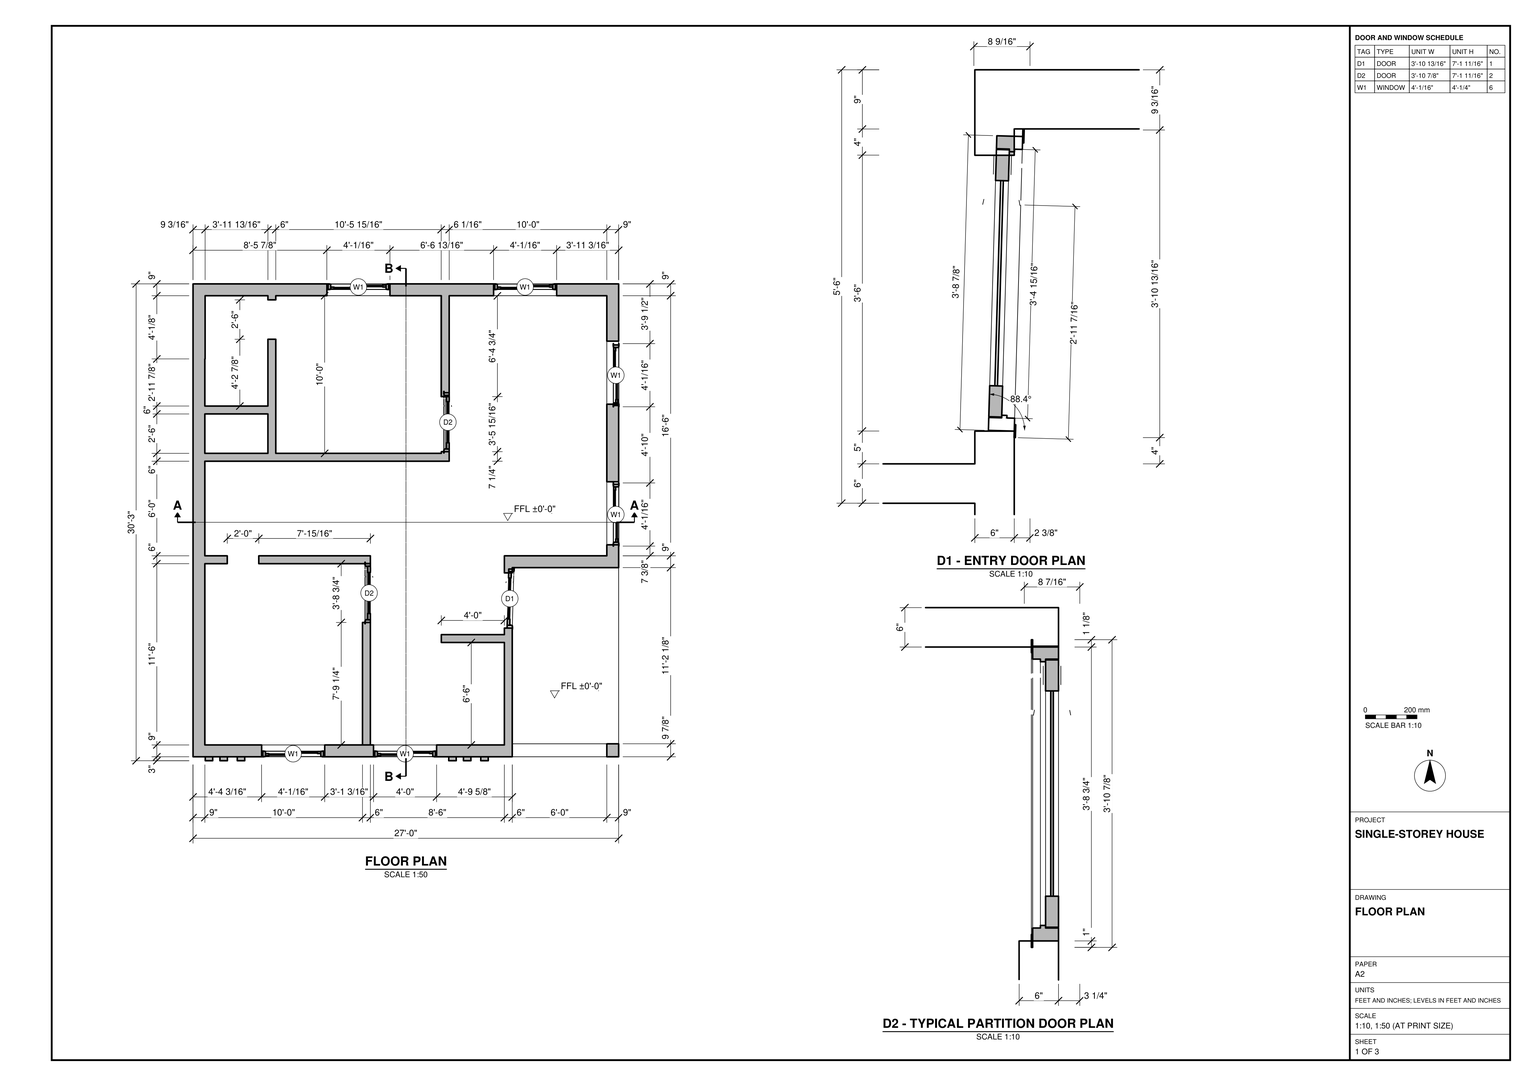
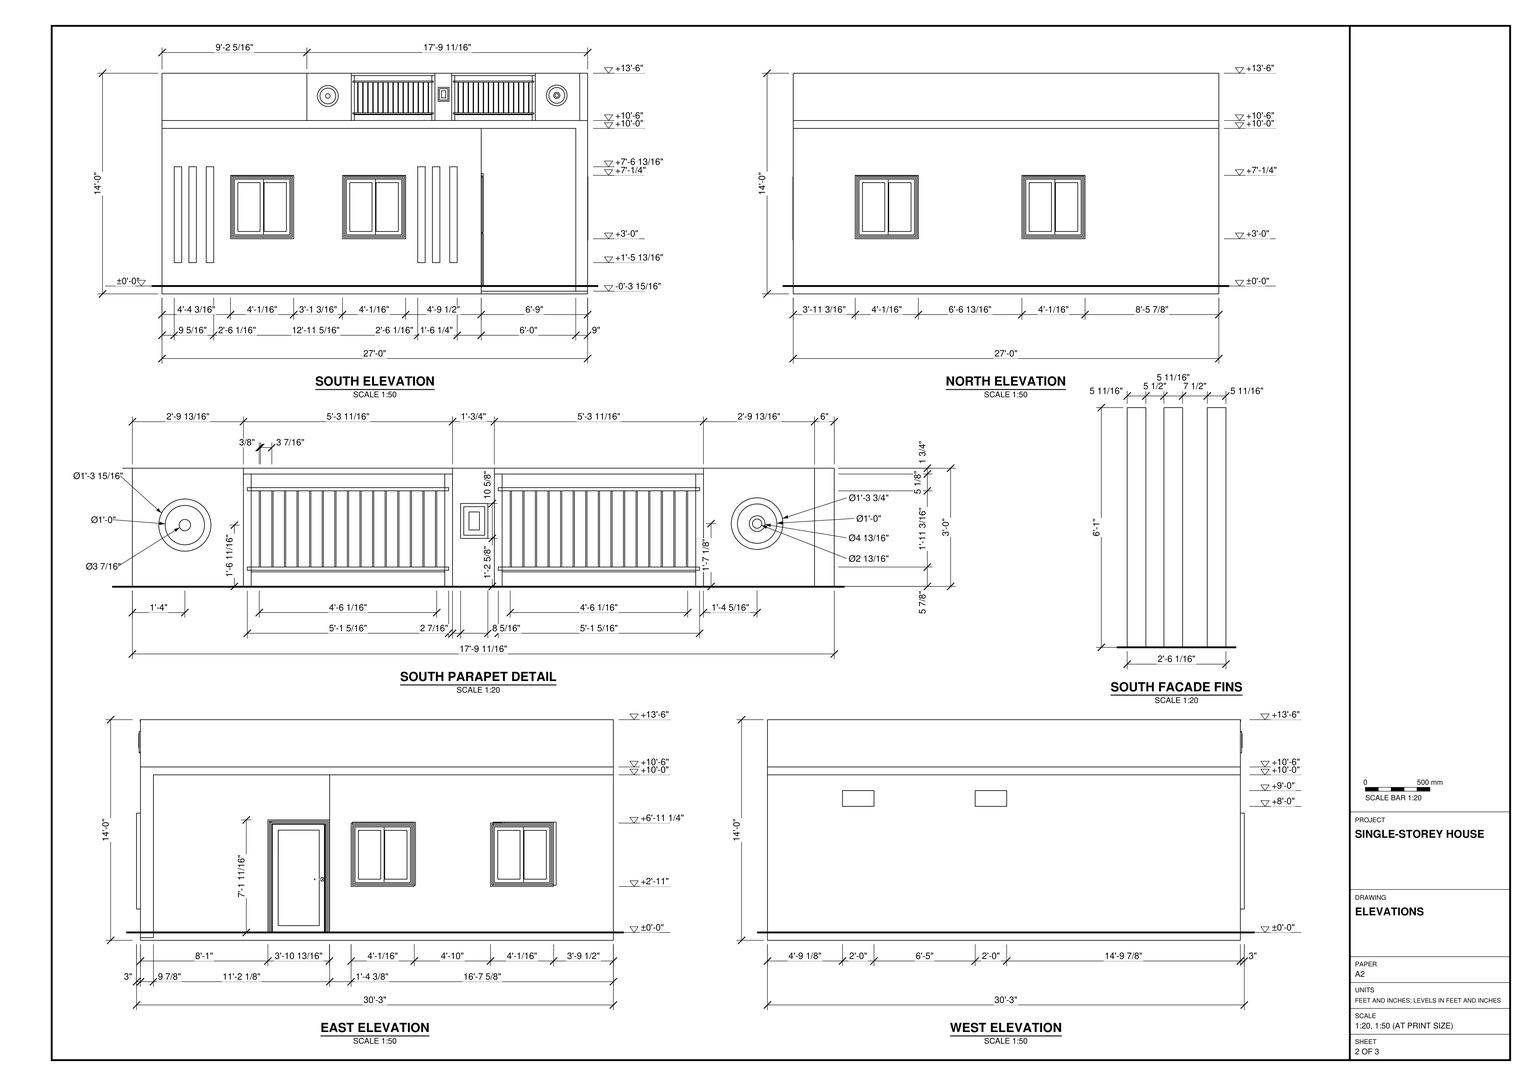
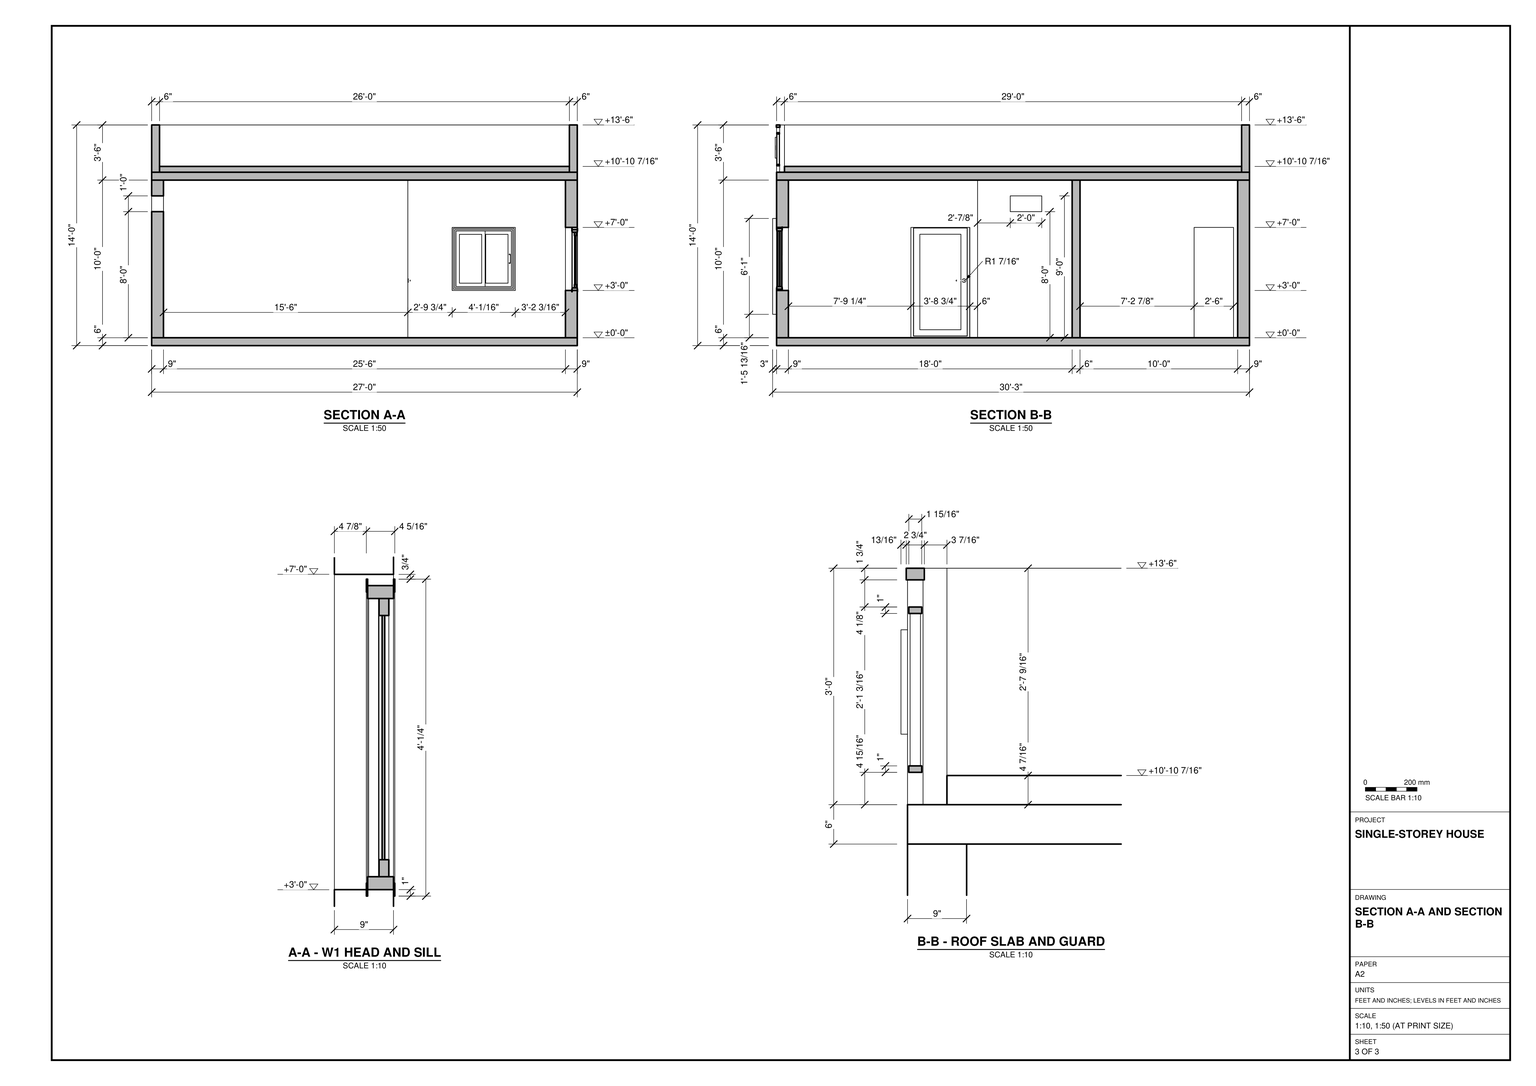
Build the single-storey house in SketchUp from task_files/diagram_01.pdf. Work in feet and inches. Set the finished floor at ±0'-0". The overall model measures 27'-3/16" east to west, 30'-3" north to south and 14'-0" from the underside of the floor slab to the top of the parapet.

Use the floor plan to set out the 9" main exterior walls and 6" partitions, following the thickness changes at the entry. Leave the southeast corner open beneath the roof, with a corner post and an entry door in the east-facing wall of the recess. Match the internal wall runs, passage gaps and two partition doors. Fit the sliding windows in pairs on the south, north and east walls, and include the two small high openings on the west wall. Use the enlarged details for the door frames, window heads and sills.

Model the floor slab, flat roof slab and perimeter parapet to the sections. On the south elevation, place the vertical fins on either side of the window pair. Above them, follow the parapet detail for the barred panels, central rectangular relief and circular end motifs. Leave the rooms unfurnished as drawn. Any decor or loose items may be suitable library components.

Keep walls, slabs and roof separate as groups or components, treat any furniture or joinery piece separately, and use components for repeated parts. Save one SketchUp model as output_files/single_storey_house_with_a_recessed_entry_and_parapet.skp.

# SketchUp Ruby script. Lengths in inches.
U = 1.inch
M = Sketchup.active_model
def pt(a) = Geom::Point3d.new(a.map { |v| v * U })
def face(e, loops, mat)
  f = e.add_face(loops[0].map { |a| pt(a) })
  loops[1..].each { |l| e.add_face(l.map { |a| pt(a) }).erase! }
  f.material = f.back_material = mat if mat
  f
end
# faces: each face lists its corners as indices into pts; further lists are holes
def faces(e, pts, list, mat = nil) = list.each { |f| face(e, (f[0].is_a?(Array) ? f : [f]).map { |l| l.map { |i| pts[i] } }, mat) }
# xy, xz, yz: faces in a plane at the given z, y or x. An outline is a flat list of corners, or four numbers for a rectangle; further outlines are holes
def ring(l) = l.size == 4 ? [[l[0], l[1]], [l[2], l[1]], [l[2], l[3]], [l[0], l[3]]] : l.each_slice(2).to_a
def flat(e, list, mat, &to3) = list.each { |f| face(e, (f[0].is_a?(Array) ? f : [f]).map { |l| ring(l).map { |u, v| to3.(u, v) } }, mat) }
def xy(e, z, list, mat = nil) = flat(e, list, mat) { |x, y| [x, y, z] }
def xz(e, y, list, mat = nil) = flat(e, list, mat) { |x, z| [x, y, z] }
def yz(e, x, list, mat = nil) = flat(e, list, mat) { |y, z| [x, y, z] }
def lines(e, pts, list) = list.each { |a, b| e.add_line(pt(pts[a]), pt(pts[b])) }
# prism: a flat outline (further loops are holes) pulled along v
def prism(e, loops, v, mat = nil)
  f = face(e, loops, mat); d = Geom::Vector3d.new(v.map { |x| x * U })
  f.pushpull(f.normal.samedirection?(d) ? d.length : -d.length)
end
def box(e, o, s, mat = nil) = prism(e, [[o, [o[0] + s[0], o[1], o[2]], [o[0] + s[0], o[1] + s[1], o[2]], [o[0], o[1] + s[1], o[2]]]], [0, 0, s[2]], mat)
def at(x, y, z, deg = 0) = Geom::Transformation.translation(pt([x, y, z])) * Geom::Transformation.rotation(ORIGIN, Z_AXIS, deg.degrees)
def axes(o, x, y, z) = Geom::Transformation.new([*x, 0, *y, 0, *z, 0, *pt(o).to_a, 1])
def part(name) = M.definitions.add(name)
# library, detail: a bought-in or finely detailed component or shape, given as its bounding box
def library(name, o, s) = part(name).tap { |d| box(d.entities, o, s) }
def detail(e, o, s) = box(e.add_group.entities, o, s)
def put(e, d, t, mat = nil) = e.add_instance(d, t).tap { |i| i.material = mat if mat }
def group(e, t, mat = nil) = e.add_group.tap { |g| g.transformation = t; g.material = mat if mat }.entities
root = M.entities
M.materials.add("[Color A02]").color = [255, 153, 153]
M.materials.add("[Formica Graystone]").color = [149, 146, 135]
M.materials.add("[Metal Corrugated Shiny]").color = [193, 193, 193]
M.materials.add("[Quartz Light Brown]").color = [199, 184, 152]
M.materials.add("[Stone Marble]").color = [143, 138, 136]
M.materials.add("[Tile Limestone Multi]").color = [199, 173, 118]
M.materials.add("[Wood Bamboo]").color = [177, 105, 43]
M.materials.add("wall").color = [255, 255, 255]
c1 = library("Single Door",[-0.98,-1.27,0],[46.84,8.45,85.7])
c2 = library("Sliding Window",[-0.98,-0.2,-0.98],[48.05,4.66,48.26])
c3 = part("Union")
xy(c3.entities,0,[[102.95,0,108.95,93.25],[24,138,108.95,144]],"wall")
xy(c3.entities,84,[[102.95,93.25,108.95,138],[0,138,24,144]],"wall")
xy(c3.entities,120,[[102.95,0,108.95,0,108.95,144,0,144,0,138,102.95,138]],"wall")
xz(c3.entities,0,[[102.95,0,108.95,120]],"wall")
xz(c3.entities,93.25,[[102.95,0,108.95,84]],"wall")
xz(c3.entities,138,[[24,0,108.95,0,108.95,84,102.95,84,102.95,120,0,120,0,84,24,84]],"wall")
xz(c3.entities,144,[[24,0,24,84,0,84,0,120,108.95,120,108.95,0]],"wall")
yz(c3.entities,0,[[138,84,144,120]],"wall")
yz(c3.entities,24,[[138,0,144,84]],"wall")
yz(c3.entities,102.95,[[0,0,0,120,138,120,138,84,93.25,84,93.25,0]],"wall")
yz(c3.entities,108.95,[[0,0,93.25,0,93.25,84,138,84,138,0,144,0,144,120,0,120]],"wall")
c4 = library("Group\#5",[0,-1,0],[33.8125,7,36])
c5 = library("Group\#6",[0,-1,0],[33.8125,7,36])
c6 = part("Group61\#1")
box(c6.entities,[230.52,30.56,126],[2.37,2.36,34.23])
c7 = part("Group63\#2")
box(c7.entities,[170.4,30.76,155.11],[61.31,1.97,0.98])
c8 = part("Group63\#1")
box(c8.entities,[169.21,30.36,160.23],[63.68,2.76,1.77])
c9 = part("Group64\#1")
box(c9.entities,[170.4,30.76,130.92],[61.31,1.97,0.99])
c10 = part("Group65\#1")
box(c10.entities,[174.03,30.95,131.91],[0.39,1.58,23.2])
box(c10.entities,[177.86,30.95,131.91],[0.4,1.58,23.2])
box(c10.entities,[181.69,30.95,131.91],[0.4,1.58,23.2])
box(c10.entities,[185.53,30.95,131.91],[0.39,1.58,23.2])
box(c10.entities,[189.36,30.95,131.91],[0.39,1.58,23.2])
box(c10.entities,[193.19,30.95,131.91],[0.39,1.58,23.2])
box(c10.entities,[197.02,30.95,131.91],[0.4,1.58,23.2])
box(c10.entities,[200.85,30.95,131.91],[0.4,1.58,23.2])
box(c10.entities,[204.6875,30.95,131.91],[0.39,1.58,23.2])
box(c10.entities,[208.52,30.95,131.91],[0.39,1.58,23.2])
box(c10.entities,[212.35,30.95,131.91],[0.39,1.58,23.2])
box(c10.entities,[216.18,30.95,131.91],[0.4,1.58,23.2])
box(c10.entities,[220.01,30.95,131.91],[0.4,1.58,23.2])
box(c10.entities,[223.85,30.95,131.91],[0.39,1.58,23.2])
box(c10.entities,[227.68,30.95,131.91],[0.39,1.58,23.2])
c11 = part("Group60\#1")
box(c11.entities,[169.21,30.56,126],[2.37,2.36,34.23])
c12 = part("Group\#8")
put(c12.entities,c6,at(-169.21,-30.36,-126))
put(c12.entities,c7,at(-169.21,-30.36,-126))
put(c12.entities,c8,at(-169.21,-30.36,-126))
put(c12.entities,c9,at(-169.21,-30.36,-126))
put(c12.entities,c10,at(-169.21,-30.36,-126))
put(c12.entities,c11,at(-169.21,-30.36,-126))
c13 = part("A$C0ee006e8.DWG\#1")
xy(c13.entities,126,[[39.67,25.74,136.58,31.74],[170.4,25.74,241.4375,31.74],[241.4375,25.74,254.05,31.74],[254.05,25.74,273.38,31.74]])
p = [[276.67,35.74,0.0625],[276.67,25.74,0.0625],[276.67,25.74,-6],[351.67,169.74,0],[357.67,169.74,0],[357.67,35.62,0],
  [357.67,162.62,0]]
lines(c13.entities,p,[[0,1],[1,2],[3,4],[5,6]])
g1 = group(c13.entities,at(33.67,25.74,120))
xy(g1,-123.93,[[315,0,324,9.875]],"[Stone Marble]")
xy(g1,0,[[[0,0,0,360,324,360,324,9.875,315,9.875,315,0],[255.85,23.27,301.24,109.83]],[[255.85,23.27,301.24,109.83],[263.44,30.86,293.65,102.24]],[263.44,30.86,293.65,102.24]],"[Stone Marble]")
xy(g1,6,[[0,0,324,360]],"[Stone Marble]")
xz(g1,0,[[315,-123.93,324,-123.93,324,6,0,6,0,0,315,0]],"[Stone Marble]")
xz(g1,9.875,[[315,-123.93,324,0]],"[Stone Marble]")
xz(g1,360,[[0,0,324,6]],"[Stone Marble]")
yz(g1,0,[[0,0,360,6]],"[Stone Marble]")
yz(g1,315,[[0,-123.93,9.875,0]],"[Stone Marble]")
yz(g1,324,[[0,-123.93,9.875,-123.93,9.875,0,360,0,360,6,0,6]],"[Stone Marble]")
g2 = group(c13.entities,at(33.67,25.74,0),"wall")
xy(g2,0,[[[0,0,0,360,324,360,324,144,243,144,243,139.99,237,139.99,237,153,315,153,315,351,195,351,195,274.28,189,274.28,189,351,63,351,63,347.86,57,347.86,57,351,9.19,351,9.19,302.89,9,302.89,9,267,57,267,57,317.86,63,317.86,63,231,189,231,189,232.28,195,232.28,195,225,9,225,9,153,26.05,153,26.05,147,9,147,9,9,237,9,237,87,189,87,189,93,237,93,237,97.99,243,97.99,243,0],[9,231,57,261]]],"[Formica Graystone]")
xy(g2,36,[[52.24,0,100.24,9],[137.41,0,185.41,9],[315,161.37,324,209.37],[315,268.43,324,316.43],[101.91,351,149.91,360],
  [228.81,351,276.81,360]],"[Formica Graystone]")
xy(g2,84,[[52.24,0,100.24,9],[137.41,0,185.41,9],[237,97.99,243,139.99],[315,161.37,324,209.37],[188.91,232.28,195,274.18],
  [315,268.43,324,316.43],[57,317.86,63,347.86],[101.91,351,149.91,360],[228.81,351,276.81,360]],"[Formica Graystone]")
xy(g2,96,[[0,177.88,9,201.88],[0,278.89,9,302.89]],"[Formica Graystone]")
xy(g2,108,[[0,177.88,9,201.88],[0,278.89,9,302.89]],"[Formica Graystone]")
xy(g2,120,[[[0,0,243,0,243,144,324,144,324,360,0,360],[9,9,9,147,26.05,147,26.05,153,9,153,9,225,195,225,195,274.18,188.91,274.18,188.91,232.28,189,232.28,189,231,63,231,63,351,189,351,189,274.28,195,274.28,195,351,315,351,315,153,237,153,237,93,189,93,189,87,237,87,237,9],[9,267,9,302.89,9.19,302.89,9.19,351,57,351,57,267],[9,231,57,261]]],"[Formica Graystone]")
xz(g2,0,[[[0,0,243,120],[137.41,36,185.41,84],[52.24,36,100.24,84]]],"[Formica Graystone]")
xz(g2,9,[[[9,0,237,120],[52.24,36,100.24,84],[137.41,36,185.41,84]]],"[Formica Graystone]")
xz(g2,87,[[189,0,237,120]],"[Formica Graystone]")
xz(g2,93,[[189,0,237,120]],"[Formica Graystone]")
xz(g2,97.99,[[237,0,243,84]],"[Formica Graystone]")
xz(g2,139.99,[[237,0,243,84]],"[Formica Graystone]")
xz(g2,144,[[243,0,324,120]],"[Formica Graystone]")
xz(g2,147,[[9,0,26.05,120]],"[Formica Graystone]")
xz(g2,153,[[9,0,26.05,120],[237,0,315,120]],"[Formica Graystone]")
xz(g2,161.37,[[315,36,324,84]],"[Formica Graystone]")
xz(g2,177.88,[[0,96,9,108]],"[Formica Graystone]")
xz(g2,201.88,[[0,96,9,108]],"[Formica Graystone]")
xz(g2,209.37,[[315,36,324,84]],"[Formica Graystone]")
xz(g2,225,[[9,0,195,120]],"[Formica Graystone]")
xz(g2,231,[[9,0,57,120],[63,0,189,120]],"[Formica Graystone]")
xz(g2,232.28,[[189,0,195,84],[188.91,84,189,120]],"[Formica Graystone]")
xz(g2,261,[[9,0,57,120]],"[Formica Graystone]")
xz(g2,267,[[9,0,57,120]],"[Formica Graystone]")
xz(g2,268.43,[[315,36,324,84]],"[Formica Graystone]")
xz(g2,274.18,[[188.91,0,195,84]],"[Formica Graystone]")
xz(g2,274.28,[[189,0,195,120]],"[Formica Graystone]")
xz(g2,278.89,[[0,96,9,108]],"[Formica Graystone]")
xz(g2,302.89,[[9,0,9.19,120],[0,96,9,108]],"[Formica Graystone]")
xz(g2,316.43,[[315,36,324,84]],"[Formica Graystone]")
xz(g2,317.86,[[57,0,63,84]],"[Formica Graystone]")
xz(g2,347.86,[[57,0,63,84]],"[Formica Graystone]")
xz(g2,351,[[9.19,0,57,120],[[63,0,189,120],[101.91,36,149.91,84]],[[195,0,315,120],[228.81,36,276.81,84]]],"[Formica Graystone]")
xz(g2,360,[[[0,0,324,120],[228.81,36,276.81,84],[101.91,36,149.91,84]]],"[Formica Graystone]")
yz(g2,0,[[[0,0,360,120],[278.89,96,302.89,108],[177.88,96,201.88,108]]],"[Formica Graystone]")
yz(g2,9,[[9,0,147,120],[[153,0,225,120],[177.88,96,201.88,108]],[231,0,261,120],[267,0,302.89,0,302.89,96,278.89,96,278.89,108,302.89,108,302.89,120,267,120]],"[Formica Graystone]")
yz(g2,9.19,[[302.89,0,351,120]],"[Formica Graystone]")
yz(g2,26.05,[[147,0,153,120]],"[Formica Graystone]")
yz(g2,52.24,[[0,36,9,84]],"[Formica Graystone]")
yz(g2,57,[[231,0,261,120],[267,0,267,120,351,120,351,0,347.86,0,347.86,84,317.86,84,317.86,0]],"[Formica Graystone]")
yz(g2,63,[[231,0,317.86,0,317.86,84,347.86,84,347.86,0,351,0,351,120,231,120]],"[Formica Graystone]")
yz(g2,100.24,[[0,36,9,84]],"[Formica Graystone]")
yz(g2,101.91,[[351,36,360,84]],"[Formica Graystone]")
yz(g2,137.41,[[0,36,9,84]],"[Formica Graystone]")
yz(g2,149.91,[[351,36,360,84]],"[Formica Graystone]")
yz(g2,185.41,[[0,36,9,84]],"[Formica Graystone]")
yz(g2,188.91,[[274.18,0,274.18,84,232.28,84,232.28,120,350.91,120,350.91,0]],"[Formica Graystone]")
yz(g2,189,[[87,0,93,120],[231,0,232.28,120],[274.28,0,351,120]],"[Formica Graystone]")
yz(g2,195,[[225,0,232.28,0,232.28,84,274.18,84,274.18,0,274.28,0,274.28,120,225,120],[274.28,0,351,120]],"[Formica Graystone]")
yz(g2,228.81,[[351,36,360,84]],"[Formica Graystone]")
yz(g2,237,[[9,0,87,120],[93,0,93,120,153,120,153,0,139.99,0,139.99,84,97.99,84,97.99,0]],"[Formica Graystone]")
yz(g2,243,[[0,0,97.99,0,97.99,84,139.99,84,139.99,0,144,0,144,120,0,120]],"[Formica Graystone]")
yz(g2,276.81,[[351,36,360,84]],"[Formica Graystone]")
yz(g2,315,[[[153,0,351,120],[161.37,36,209.37,84],[268.43,36,316.43,84]]],"[Formica Graystone]")
yz(g2,324,[[[144,0,360,120],[161.37,36,209.37,84],[268.43,36,316.43,84]]],"[Formica Graystone]")
put(c13.entities,c3,at(59.72,34.74,0))
g3 = group(c13.entities,at(33.67,25.74,126),"[Quartz Light Brown]")
xy(g3,0,[[0,0,110.28,0,110.28,6,6,6,6,354,318,354,318,0,324,0,324,360,0,360],[110.28,0,136.73,6],[136.73,0,318,6]])
xy(g3,36,[[0,0,110.28,0,110.28,6,6,6,6,354,318,354,318,0,324,0,324,360,0,360]])
xz(g3,0,[[0,0,110.28,36],[318,0,324,36]])
xz(g3,6,[[6,0,110.28,36]])
xz(g3,354,[[6,0,318,36]])
xz(g3,360,[[0,0,324,36]])
yz(g3,0,[[0,0,360,36]])
yz(g3,6,[[6,0,354,36]])
yz(g3,110.28,[[0,0,6,36]])
yz(g3,318,[[0,0,6,36],[6,0,354,36]])
yz(g3,324,[[0,0,360,36]])
p = [[107.91,0,0],[107.91,-0.06,0]]
lines(g3,p,[[0,1]])
put(g3,c4,at(110.28,0,0),"[Color A02]")
put(g3,c5,at(284.1875,0,0),"[Color A02]")
g4 = group(g3,at(6,6,0))
prism(g4,[[[0,348,0],[312,348,0],[312,0,0],[130.73,0,0],[104.28,0,0],[0,0,0]]],[0,0,4.4375])
put(c13.entities,c12,at(177.76,25.54,126),"[Metal Corrugated Shiny]")
put(c13.entities,c12,at(254.18,25.54,126),"[Metal Corrugated Shiny]")
g5 = group(c13.entities,at(33.67,25.74,-6),"[Tile Limestone Multi]")
xy(g5,0,[[0,0,324,360]])
xy(g5,2.07,[[243,0,324,9.875]])
xy(g5,6,[[0,0,243,0,243,9.875,324,9.875,324,360,0,360]])
xz(g5,0,[[0,0,243,6],[243,0,324,2.07]])
xz(g5,9.875,[[243,2.07,324,6]])
xz(g5,360,[[0,0,324,6]])
yz(g5,0,[[0,0,360,6]])
yz(g5,243,[[0,2.07,9.875,6]])
yz(g5,324,[[0,0,360,0,360,6,9.875,6,9.875,2.07,0,2.07]])
p = [[243,0,6],[243,0,6.0625]]
lines(g5,p,[[0,1]])
c14 = part("Timber post")
box(c14.entities,[0,-3,0],[5.6875,3,73],"[Wood Bamboo]")
xy(root,126,[[207.77,3,220.51,9]],"[Color A02]")
xy(root,140.625,[[210.22,1.6875,218.53,3]],"[Color A02]")
xy(root,141.59,[[211.18,1.6875,217.57,3]],"[Color A02]")
xy(root,143.19,[[212.78,1.8125,215.97,3]],"[Color A02]")
xy(root,148.69,[[212.78,1.8125,215.97,3]],"[Color A02]")
xy(root,150.29,[[211.18,1.6875,217.57,3]],"[Color A02]")
xy(root,151.25,[[210.22,1.6875,218.53,3]],"[Color A02]")
xy(root,162,[[207.77,3,220.51,9]],"[Color A02]")
xz(root,1.6875,[[[210.22,140.625,218.53,151.25],[211.18,141.59,217.57,150.29]]],"[Color A02]")
xz(root,1.8125,[[212.78,143.19,215.97,148.69]],"[Color A02]")
xz(root,3,[[[207.77,126,220.51,162],[210.22,140.625,218.53,151.25]],[[211.18,141.59,217.57,150.29],[212.78,143.19,215.97,148.69]]],"[Color A02]")
xz(root,9,[[207.77,126,220.51,162]],"[Color A02]")
yz(root,207.77,[[3,126,9,162]],"[Color A02]")
yz(root,210.22,[[1.6875,140.625,3,151.25]],"[Color A02]")
yz(root,211.18,[[1.6875,141.59,3,150.29]],"[Color A02]")
yz(root,212.78,[[1.8125,143.19,3,148.69]],"[Color A02]")
yz(root,215.97,[[1.8125,143.19,3,148.69]],"[Color A02]")
yz(root,217.57,[[1.6875,141.59,3,150.29]],"[Color A02]")
yz(root,218.53,[[1.6875,140.625,3,151.25]],"[Color A02]")
yz(root,220.51,[[3,126,9,162]],"[Color A02]")
p = [[136.73,9,126],[136.73,3,126]]
lines(root,p,[[0,1]])
put(root,c1,at(243,100.99,0,88.363))
put(root,c1,axes([191.0625,235.28,84],[0,1,0],[1,0,0],[0,0,-1]))
put(root,c2,at(324,164.37,36,90))
put(root,c2,at(148.93,362.8,36.98,-180))
put(root,c2,at(275.82,362.8,36.98,-180))
put(root,c2,at(324,270.44,36,90))
put(root,c2,at(53.17,3.2,36.98))
put(root,c2,at(138.39,3.2,36.98))
put(root,c1,axes([131.0625,105.25,84],[0,1,0],[1,0,0],[0,0,-1]))
put(root,c13,at(-33.67,-22.74,0))
g6 = group(root,at(9.3,0,17.82))
put(g6,c14,at(185.37,3,0),"[Wood Bamboo]")
put(g6,c14,at(196.55,3,0),"[Wood Bamboo]")
put(g6,c14,at(0,3,0))
put(g6,c14,at(209.74,3,0))
put(g6,c14,at(24.375,3,0))
put(g6,c14,at(11.1875,3,0))
